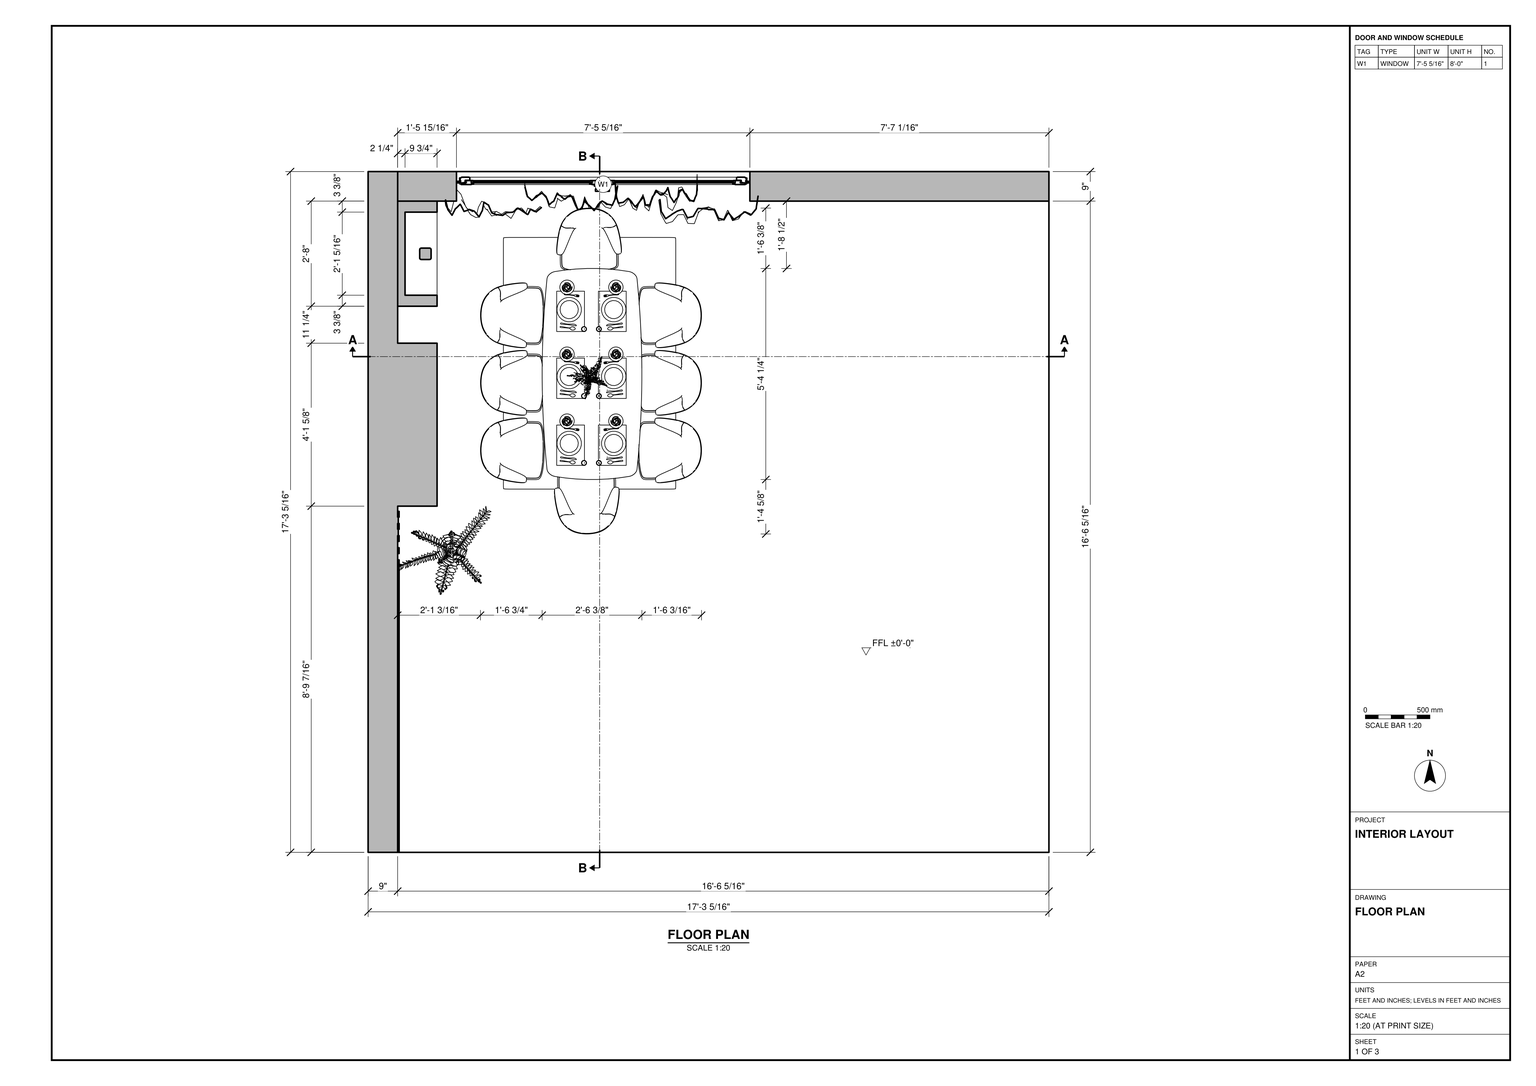
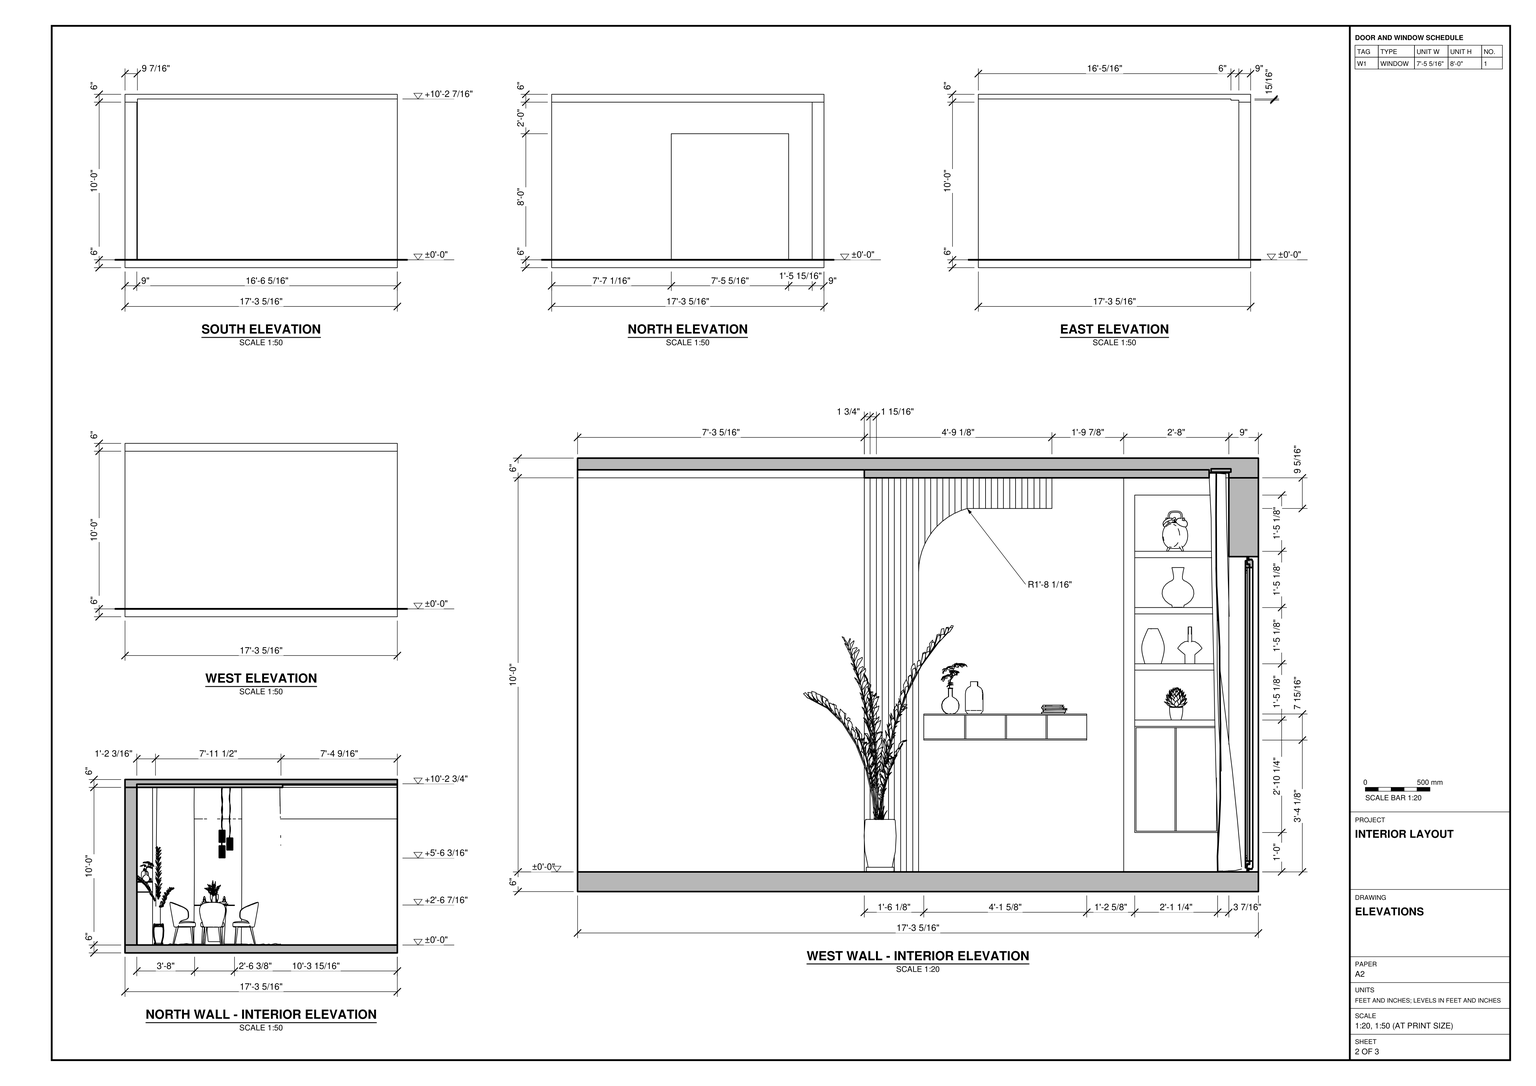
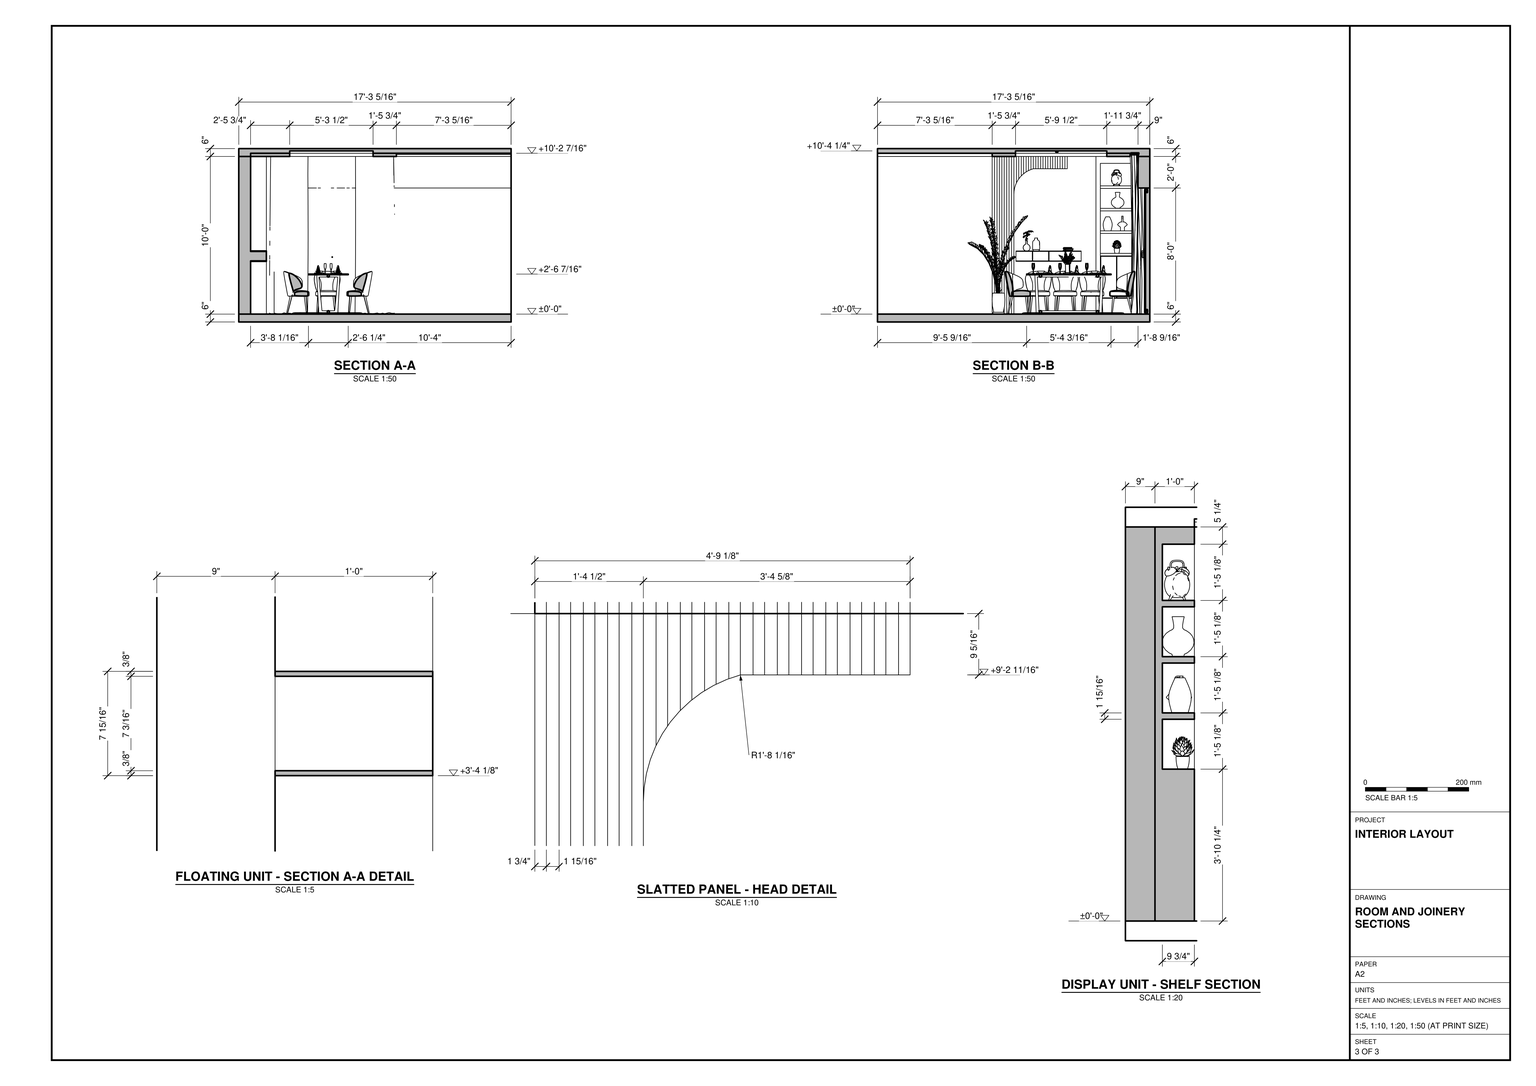
Build the dining room in SketchUp using task_files/diagram_01.pdf. Work in feet and inches. The overall footprint is 17'-3 5/16" by 17'-3 5/16", the overall height is 11'-0", and the finished floor level is ±0'-0". Model the floor slab, the 9" north and west walls and the overhead slab. Follow the sections for the slab thicknesses and changes in the ceiling profile. Leave the south and east sides open as drawn.

Place the floor-height window and curtains near the west end of the north wall. Set the dining table with its long axis running north–south in front of the window. Arrange three chairs along each long side and one at each end, with the rug beneath the setting and pendant lighting above it.

Use the west wall elevation and joinery details to model the vertical slats and their curved return into a horizontal head. Fit the shallow floating unit beside the slats and the tall display unit nearer the window. Include the display shelves, lower cabinet and loose items in the positions shown. Decor and loose items may be any suitable library components.

Keep the walls, slabs and each furniture or joinery piece in separate groups or components, and use components for repeated parts. Save one SketchUp model as output_files/dining_room_with_slatted_panelling_and_display_joinery.skp.

# SketchUp Ruby script. Lengths in inches.
U = 1.inch
M = Sketchup.active_model
def pt(a) = Geom::Point3d.new(a.map { |v| v * U })
def face(e, loops, mat)
  f = e.add_face(loops[0].map { |a| pt(a) })
  loops[1..].each { |l| e.add_face(l.map { |a| pt(a) }).erase! }
  f.material = f.back_material = mat if mat
  f
end
# faces: each face lists its corners as indices into pts; further lists are holes
def faces(e, pts, list, mat = nil) = list.each { |f| face(e, (f[0].is_a?(Array) ? f : [f]).map { |l| l.map { |i| pts[i] } }, mat) }
# xy, xz, yz: faces in a plane at the given z, y or x. An outline is a flat list of corners, or four numbers for a rectangle; further outlines are holes
def ring(l) = l.size == 4 ? [[l[0], l[1]], [l[2], l[1]], [l[2], l[3]], [l[0], l[3]]] : l.each_slice(2).to_a
def flat(e, list, mat, &to3) = list.each { |f| face(e, (f[0].is_a?(Array) ? f : [f]).map { |l| ring(l).map { |u, v| to3.(u, v) } }, mat) }
def xy(e, z, list, mat = nil) = flat(e, list, mat) { |x, y| [x, y, z] }
def xz(e, y, list, mat = nil) = flat(e, list, mat) { |x, z| [x, y, z] }
def yz(e, x, list, mat = nil) = flat(e, list, mat) { |y, z| [x, y, z] }
def lines(e, pts, list) = list.each { |a, b| e.add_line(pt(pts[a]), pt(pts[b])) }
# prism: a flat outline (further loops are holes) pulled along v
def prism(e, loops, v, mat = nil)
  f = face(e, loops, mat); d = Geom::Vector3d.new(v.map { |x| x * U })
  f.pushpull(f.normal.samedirection?(d) ? d.length : -d.length)
end
def box(e, o, s, mat = nil) = prism(e, [[o, [o[0] + s[0], o[1], o[2]], [o[0] + s[0], o[1] + s[1], o[2]], [o[0], o[1] + s[1], o[2]]]], [0, 0, s[2]], mat)
def at(x, y, z, deg = 0) = Geom::Transformation.translation(pt([x, y, z])) * Geom::Transformation.rotation(ORIGIN, Z_AXIS, deg.degrees)
def axes(o, x, y, z) = Geom::Transformation.new([*x, 0, *y, 0, *z, 0, *pt(o).to_a, 1])
def part(name) = M.definitions.add(name)
# library, detail: a bought-in or finely detailed component or shape, given as its bounding box
def library(name, o, s) = part(name).tap { |d| box(d.entities, o, s) }
def detail(e, o, s) = box(e.add_group.entities, o, s)
def put(e, d, t, mat = nil) = e.add_instance(d, t).tap { |i| i.material = mat if mat }
def group(e, t, mat = nil) = e.add_group.tap { |g| g.transformation = t; g.material = mat if mat }.entities
root = M.entities
M.materials.add("Emissive").color = [224, 222, 181]
M.materials.add("[Color M01]").color = [226, 226, 226]
M.materials.add("[Color M03]").color = [179, 160, 140]
M.materials.add("[Color M05]").color = [114, 114, 114]
M.materials.add("[Wood Floor]").color = [155, 105, 61]
c1 = library("Window 46-12",[-37.28,-2.15,0],[74.56,4.3,92.91])
c2 = library("Curtains 001",[-91.88,-6.87,0.16],[183.71,15.03,109.46])
c3 = library("Dining Table",[-4.14,-4.14,0],[95.74,137.21,49.0625])
c4 = library("Rug 293 007",[-90.2,-61.78,-0.71],[180.4,123.56,1.82])
c5 = library("Potted Plant 02",[-16.98,-19.78,0],[30.04,38.68,37.52])
c6 = library("Vase 111-18",[-4.54,-2.8,0.01],[10.64,7.87,15.5])
c7 = library("Vase 010",[-2.69,-2.69,0.01],[5.38,5.38,9.84])
c8 = library("Vase 20-10",[-4.83,-4.83,0],[9.66,9.66,14.63])
c9 = library("Ornamental Vase 001",[-3.84,-3.66,0],[7.68,7.32,10.13])
c10 = library("Vase 298 004 008",[-3.43,-3.43,-0.03],[6.86,6.87,9.09])
c11 = library("Alarm Clock 114 007",[-2.86,-1.17,0.01],[5.71,2.99,7.86])
c12 = library("Potted Plant 50-23",[-3.4,-3.5,0],[6.8,7,9.93])
c13 = library("Books 193 006",[-5.22,-3.55,0],[10.44,7.83,2.69])
c14 = library("Pendant 35-41",[-5.93,-5.84,-58.05],[11.88,11.67,58.05])
xy(root,-6,[[0,0,207.3125,207.3125]])
xy(root,0,[[0,0,0,207.3125,9,207.3125,9,102.08,9.1875,102.08,9.1875,100.14,9,100.14,9,98.39,9.1875,98.39,9.1875,96.45,9,96.45,9,0],[9,0,9.4375,87.3125],[9,87.3125,9.4375,89.07],[9,91,9.4375,92.76],[9,94.7,9.4375,96.45],
  [9,98.39,9.4375,100.14],[9,102.08,9.4375,103.84],[9,166.3,21,198.3125],[9,198.3125,26.91,207.3125],[116.25,198.3125,207.3125,207.3125]])
xy(root,0,[[9.4375,0,207.3125,0,207.3125,198.3125,116.25,198.3125,116.25,207.3125,26.91,207.3125,26.91,198.3125,21,198.3125,21,166.3,9,166.3,9,103.84,9.4375,103.84,9.4375,102.08,9.1875,102.08,9.1875,100.14,9.4375,100.14,9.4375,98.39,9.1875,98.39,9.1875,96.45,9.4375,96.45,9.4375,94.7,9,94.7,9,92.76,9.4375,92.76,9.4375,91,9,91,9,89.07,9.4375,89.07]],"[Color M05]")
xy(root,40.14,[[9,105.42,10,155.05],[10,105.42,21,155.05]])
xy(root,40.52,[[9,105.42,21,155.05]])
xy(root,46.25,[[11.25,169.66,21,194.96]])
xy(root,47.7,[[9,105.42,21,155.05]])
xy(root,48.08,[[9,105.42,21,155.05]])
xy(root,61.4375,[[12.25,169.66,21,194.96]])
xy(root,61.4375,[[11.25,169.66,12.25,194.96]],"Emissive")
xy(root,63.375,[[11.25,169.66,21,194.96]],"[Color M05]")
xy(root,78.5625,[[12.25,169.66,21,194.96]])
xy(root,78.5625,[[11.25,169.66,12.25,194.96]],"Emissive")
xy(root,80.5,[[11.25,169.66,21,194.96]])
xy(root,95.6875,[[11.25,169.66,12.25,194.96]],"Emissive")
xy(root,95.6875,[[12.25,169.66,21,194.96]],"[Color M05]")
xy(root,96,[[26.91,198.3125,116.25,207.3125]])
xy(root,97.625,[[11.25,169.66,21,194.96]])
xy(root,110.66,[[9,118.6,9.1875,120.54],[9,120.54,9.4375,122.29],[9,122.29,9.1875,124.23],[9,124.23,9.4375,125.99],[9,125.99,9.1875,127.92],
  [9,127.92,9.4375,129.68],[9,129.68,9.1875,131.61],[9,131.61,9.4375,133.37],[9,133.37,9.1875,135.3],[9,135.3,9.4375,137.0625],
  [9,137.0625,9.1875,139],[9,139,9.4375,140.75],[9,140.75,9.1875,142.6875],[9,142.6875,9.4375,144.44]],"Emissive")
xy(root,114.75,[[11.25,169.66,12.25,194.96]],"Emissive")
xy(root,114.75,[[12.25,169.66,21,194.96]],"[Color M05]")
xy(root,120,[[0,0,0,207.3125,9,207.3125,9,142.6875,9.1875,142.6875,9.1875,140.75,9,140.75,9,139,9.1875,139,9.1875,137.0625,9,137.0625,9,135.3,9.1875,135.3,9.1875,133.37,9,133.37,9,131.61,9.1875,131.61,9.1875,129.68,9,129.68,9,127.92,9.1875,127.92,9.1875,125.99,9,125.99,9,124.23,9.1875,124.23,9.1875,122.29,9,122.29,9,120.54,9.1875,120.54,9.1875,118.6,9,118.6,9,116.85,9.1875,116.85,9.1875,114.91,9,114.91,9,113.15,9.1875,113.15,9.1875,111.22,9,111.22,9,109.46,9.1875,109.46,9.1875,107.53,9,107.53,9,105.77,9.1875,105.77,9.1875,103.84,9,103.84,9,102.08,9.1875,102.08,9.1875,100.14,9,100.14,9,98.39,9.1875,98.39,9.1875,96.45,9,96.45,9,0],[9,0,9.4375,87.3125],[9,87.3125,9.4375,89.07],[9,91,9.4375,92.76],[9,94.7,9.4375,96.45],
  [9,98.39,9.4375,100.14],[9,102.08,9.4375,103.84],[9,105.77,9.4375,107.53],[9,109.46,9.4375,111.22],[9,113.15,9.4375,114.91],
  [9,116.85,9.4375,118.6],[9,120.54,9.4375,122.29],[9,124.23,9.4375,125.99],[9,127.92,9.4375,129.68],[9,131.61,9.4375,133.37],
  [9,135.3,9.4375,137.0625],[9,139,9.4375,140.75],[9,142.6875,9.4375,144.44],[9,166.3,21,198.3125],[9,198.3125,207.3125,207.3125]])
xy(root,120,[[[9.4375,87.3125,9.4375,89.07,9,89.07,9,91,9.4375,91,9.4375,92.76,9,92.76,9,94.7,9.4375,94.7,9.4375,96.45,9.1875,96.45,9.1875,98.39,9.4375,98.39,9.4375,100.14,9.1875,100.14,9.1875,102.08,9.4375,102.08,9.4375,103.84,9.1875,103.84,9.1875,105.77,9.4375,105.77,9.4375,107.53,9.1875,107.53,9.1875,109.46,9.4375,109.46,9.4375,111.22,9.1875,111.22,9.1875,113.15,9.4375,113.15,9.4375,114.91,9.1875,114.91,9.1875,116.85,9.4375,116.85,9.4375,118.6,9.1875,118.6,9.1875,120.54,9.4375,120.54,9.4375,122.29,9.1875,122.29,9.1875,124.23,9.4375,124.23,9.4375,125.99,9.1875,125.99,9.1875,127.92,9.4375,127.92,9.4375,129.68,9.1875,129.68,9.1875,131.61,9.4375,131.61,9.4375,133.37,9.1875,133.37,9.1875,135.3,9.4375,135.3,9.4375,137.0625,9.1875,137.0625,9.1875,139,9.4375,139,9.4375,140.75,9.1875,140.75,9.1875,142.6875,9.4375,142.6875,9.4375,144.44,9,144.44,9,166.3,21,166.3,21,192.3125,120,192.3125,120,87.3125],[38.76,105.07,102.24,174.55]]],"[Color M01]")
xy(root,121.5,[[21,192.3125,207.3125,198.3125]])
xy(root,122.4375,[[9.4375,0,120,87.3125],[120,0,207.3125,192.3125],[[9.4375,87.3125,120,87.3125,120,192.3125,21,192.3125,21,166.3,9,166.3,9,144.44,9.4375,144.44,9.4375,142.6875,9.1875,142.6875,9.1875,140.75,9,140.75,9,139,9.1875,139,9.1875,137.0625,9,137.0625,9,135.3,9.1875,135.3,9.1875,133.37,9,133.37,9,131.61,9.1875,131.61,9.1875,129.68,9,129.68,9,127.92,9.1875,127.92,9.1875,125.99,9,125.99,9,124.23,9.1875,124.23,9.1875,122.29,9,122.29,9,120.54,9.1875,120.54,9.1875,118.6,9,118.6,9,116.85,9.1875,116.85,9.1875,114.91,9,114.91,9,113.15,9.1875,113.15,9.1875,111.22,9,111.22,9,109.46,9.1875,109.46,9.1875,107.53,9,107.53,9,105.77,9.1875,105.77,9.1875,103.84,9,103.84,9,102.08,9.1875,102.08,9.1875,100.14,9,100.14,9,98.39,9.1875,98.39,9.1875,96.45,9,96.45,9,89.07,9.4375,89.07],[38.76,105.07,102.24,174.55]]])
xy(root,124.25,[[38.76,105.07,102.24,174.55]])
xy(root,126,[[0,0,207.3125,207.3125]])
xz(root,0,[[0,-6,207.3125,0],[0,0,9,120],[9,0,9.4375,120],[9.4375,0,207.3125,122.4375],[0,120,9.4375,120,9.4375,122.4375,207.3125,122.4375,207.3125,126,0,126]])
xz(root,87.3125,[[9,0,9.4375,120],[9.4375,120,120,122.4375]])
xz(root,89.07,[[9,120,9.4375,122.4375]])
xz(root,89.07,[[9,0,9.4375,120]],"[Wood Floor]")
xz(root,91,[[9,0,9.4375,120]],"[Wood Floor]")
xz(root,92.76,[[9,0,9.4375,120]],"[Wood Floor]")
xz(root,94.7,[[9,0,9.4375,120]],"[Wood Floor]")
xz(root,96.45,[[9,0,9.1875,120],[9,120,9.1875,122.4375]])
xz(root,96.45,[[9.1875,0,9.4375,120]],"[Wood Floor]")
xz(root,98.39,[[9,0,9.1875,120],[9,120,9.1875,122.4375]])
xz(root,98.39,[[9.1875,0,9.4375,120]],"[Wood Floor]")
xz(root,100.14,[[9,0,9.1875,120],[9,120,9.1875,122.4375]])
xz(root,100.14,[[9.1875,0,9.4375,120]],"[Wood Floor]")
xz(root,102.08,[[9,0,9.1875,120],[9,120,9.1875,122.4375]])
xz(root,102.08,[[9.1875,0,9.4375,120]],"[Wood Floor]")
xz(root,103.84,[[9,91.35,9.1875,120],[9.1875,91.35,9.4375,120],[9,120,9.1875,122.4375]])
xz(root,103.84,[[9,0,9.4375,91.35]],"[Wood Floor]")
xz(root,105.07,[[38.76,120,102.24,122.4375]])
xz(root,105.07,[[38.76,122.4375,102.24,124.25]],"Emissive")
xz(root,105.42,[[9,40.14,21,40.52],[9,47.7,21,48.08]])
xz(root,105.42,[[9,40.52,21,47.7]],"[Color M05]")
xz(root,105.77,[[9,99.91,9.1875,120],[9.1875,99.91,9.4375,120],[9,120,9.1875,122.4375]])
xz(root,107.53,[[9,102.88,9.1875,120],[9.1875,102.88,9.4375,120],[9,120,9.1875,122.4375]])
xz(root,109.46,[[9,105.25,9.1875,120],[9.1875,105.25,9.4375,120],[9,120,9.1875,122.4375]])
xz(root,111.22,[[9,106.85,9.1875,120],[9.1875,106.85,9.4375,120],[9,120,9.1875,122.4375]])
xz(root,113.15,[[9,108.24,9.1875,120],[9.1875,108.24,9.4375,120],[9,120,9.1875,122.4375]])
xz(root,114.91,[[9,109.24,9.1875,120],[9.1875,109.24,9.4375,120],[9,120,9.1875,122.4375]])
xz(root,116.85,[[9,110.08,9.1875,120],[9.1875,110.08,9.4375,120],[9,120,9.1875,122.4375]])
xz(root,118.6,[[9,110.66,9.1875,120],[9.1875,110.66,9.4375,120],[9,120,9.1875,122.4375]])
xz(root,120.54,[[9,110.66,9.1875,120],[9.1875,110.66,9.4375,120],[9,120,9.1875,122.4375]])
xz(root,122.29,[[9,110.66,9.1875,120],[9.1875,110.66,9.4375,120],[9,120,9.1875,122.4375]])
xz(root,124.23,[[9,110.66,9.1875,120],[9.1875,110.66,9.4375,120],[9,120,9.1875,122.4375]])
xz(root,125.99,[[9,110.66,9.1875,120],[9.1875,110.66,9.4375,120],[9,120,9.1875,122.4375]])
xz(root,127.92,[[9,110.66,9.1875,120],[9.1875,110.66,9.4375,120],[9,120,9.1875,122.4375]])
xz(root,129.68,[[9,110.66,9.1875,120],[9.1875,110.66,9.4375,120],[9,120,9.1875,122.4375]])
xz(root,131.61,[[9,110.66,9.1875,120],[9.1875,110.66,9.4375,120],[9,120,9.1875,122.4375]])
xz(root,133.37,[[9,110.66,9.1875,120],[9.1875,110.66,9.4375,120],[9,120,9.1875,122.4375]])
xz(root,135.3,[[9,110.66,9.1875,120],[9.1875,110.66,9.4375,120],[9,120,9.1875,122.4375]])
xz(root,137.0625,[[9,110.66,9.1875,120],[9.1875,110.66,9.4375,120],[9,120,9.1875,122.4375]])
xz(root,139,[[9,110.66,9.1875,120],[9.1875,110.66,9.4375,120],[9,120,9.1875,122.4375]])
xz(root,140.75,[[9,110.66,9.1875,120],[9.1875,110.66,9.4375,120],[9,120,9.1875,122.4375]])
xz(root,142.6875,[[9,110.66,9.1875,120],[9.1875,110.66,9.4375,120],[9.1875,120,9.4375,122.4375]])
xz(root,144.44,[[9,110.66,9.4375,120],[9,120,9.4375,122.4375]])
xz(root,155.05,[[9,40.14,21,40.52],[9,40.52,21,47.7],[9,47.7,21,48.08]])
xz(root,166.3,[[9,120,21,122.4375]])
xz(root,166.3,[[9,0,21,120]],"[Color M05]")
xz(root,169.66,[[11.25,46.25,21,61.4375],[11.25,63.375,21,78.5625],[11.25,80.5,21,95.6875],[11.25,97.625,21,114.75]])
xz(root,174.55,[[38.76,120,102.24,122.4375]])
xz(root,174.55,[[38.76,122.4375,102.24,124.25]],"Emissive")
xz(root,192.3125,[[21,120,120,121.5],[21,121.5,120,122.4375],[120,121.5,207.3125,122.4375]])
xz(root,194.96,[[11.25,46.25,21,61.4375],[11.25,63.375,21,78.5625],[11.25,80.5,21,95.6875],[11.25,97.625,21,114.75]],"[Color M05]")
xz(root,198.3125,[[9,0,21,120],[21,0,26.91,0,26.91,96,207.3125,96,207.3125,120,21,120],[116.25,0,207.3125,96],[21,120,207.3125,121.5]])
xz(root,207.3125,[[0,-6,207.3125,0],[0,0,9,120],[9,0,9,120,207.3125,120,207.3125,0,116.25,0,116.25,96,26.91,96,26.91,0],[26.91,0,116.25,96],[0,120,207.3125,126]])
yz(root,0,[[0,-6,207.3125,0],[0,0,207.3125,120],[0,120,207.3125,126]])
yz(root,9,[[0,0,87.3125,120],[87.3125,0,89.07,120],[91,0,92.76,120],[94.7,0,96.45,120],[98.39,0,100.14,120],
  [102.08,0,103.84,120],[166.3,0,198.3125,120],[198.3125,0,207.3125,120],[105.42,40.14,155.05,40.52],[105.42,47.7,155.05,48.08],
  [105.77,99.91,105.77,120,107.53,120,107.53,102.88,106.73,101.71],[109.46,105.25,109.46,120,111.22,120,111.22,106.85,110.95,106.65],[113.15,108.24,113.15,120,114.91,120,114.91,109.24,114.56,109.07],[116.85,110.08,116.85,120,118.6,120,118.6,110.66],[120.54,110.66,122.29,120],
  [124.23,110.66,125.99,120],[127.92,110.66,129.68,120],[131.61,110.66,133.37,120],[135.3,110.66,137.0625,120],[139,110.66,140.75,120],
  [142.6875,110.66,144.44,120],[89.07,120,91,122.4375],[91,120,92.76,122.4375],[92.76,120,94.7,122.4375],[94.7,120,96.45,122.4375],
  [98.39,120,100.14,122.4375],[102.08,120,103.84,122.4375],[105.77,120,107.53,122.4375],[109.46,120,111.22,122.4375],[113.15,120,114.91,122.4375],
  [116.85,120,118.6,122.4375],[120.54,120,122.29,122.4375],[124.23,120,125.99,122.4375],[127.92,120,129.68,122.4375],[131.61,120,133.37,122.4375],
  [135.3,120,137.0625,122.4375],[139,120,140.75,122.4375],[144.44,120,166.3,122.4375]])
yz(root,9,[[[103.84,0,166.3,0,166.3,120,144.44,120,144.44,110.66,118.6,110.66,116.85,110.08,116.54,109.98,114.91,109.24,114.56,109.07,113.15,108.24,112.6875,107.96,111.22,106.85,110.95,106.65,109.46,105.25,109.36,105.16,107.95,103.5,107.53,102.88,106.73,101.71,105.77,99.91,105.7,99.78,104.89,97.76,104.31,95.67,103.95,93.52,103.84,91.35],[105.42,40.14,155.05,48.08]]],"[Color M03]")
yz(root,9,[[89.07,0,91,120],[92.76,0,94.7,120]],"[Wood Floor]")
yz(root,9.1875,[[96.45,120,98.39,122.4375],[100.14,120,102.08,122.4375],[103.84,120,105.77,122.4375],[107.53,120,109.46,122.4375],[111.22,120,113.15,122.4375],
  [114.91,120,116.85,122.4375],[118.6,120,120.54,122.4375],[122.29,120,124.23,122.4375],[125.99,120,127.92,122.4375],[129.68,120,131.61,122.4375],
  [133.37,120,135.3,122.4375],[137.0625,120,139,122.4375],[140.75,120,142.6875,122.4375]])
yz(root,9.1875,[[96.45,0,98.39,120],[100.14,0,102.08,120],[103.84,91.35,103.95,93.52,104.31,95.67,104.89,97.76,105.7,99.78,105.77,99.91,105.77,120,103.84,120],[107.53,102.88,107.95,103.5,109.36,105.16,109.46,105.25,109.46,120,107.53,120],[111.22,106.85,112.6875,107.96,113.15,108.24,113.15,120,111.22,120],
  [114.91,109.24,116.54,109.98,116.85,110.08,116.85,120,114.91,120],[118.6,110.66,120.54,120],[122.29,110.66,124.23,120],[125.99,110.66,127.92,120],[129.68,110.66,131.61,120],
  [133.37,110.66,135.3,120],[137.0625,110.66,139,120],[140.75,110.66,142.6875,120]],"[Wood Floor]")
yz(root,9.4375,[[0,0,87.3125,120],[0,120,87.3125,122.4375],[87.3125,120,89.07,122.4375],[142.6875,120,144.44,122.4375]])
yz(root,9.4375,[[87.3125,0,89.07,120],[91,0,92.76,120],[94.7,0,96.45,120],[98.39,0,100.14,120],[102.08,0,103.84,120],
  [105.77,99.91,106.73,101.71,107.53,102.88,107.53,120,105.77,120],[109.46,105.25,110.95,106.65,111.22,106.85,111.22,120,109.46,120],[113.15,108.24,114.56,109.07,114.91,109.24,114.91,120,113.15,120],[116.85,110.08,118.6,110.66,118.6,120,116.85,120],[120.54,110.66,122.29,120],
  [124.23,110.66,125.99,120],[127.92,110.66,129.68,120],[131.61,110.66,133.37,120],[135.3,110.66,137.0625,120],[139,110.66,140.75,120],
  [142.6875,110.66,144.44,120]],"[Wood Floor]")
yz(root,11.25,[[169.66,46.25,194.96,61.4375],[169.66,63.375,194.96,78.5625],[169.66,80.5,194.96,95.6875],[169.66,97.625,194.96,114.75]],"[Color M05]")
yz(root,21,[[[169.66,12,194.96,44.3125],[170.06,12.4,194.5625,43.91]],[181.91,12.4,182.31,43.91],[105.42,40.14,155.05,40.52],[117.83,40.52,118.23,47.7],[130.24,40.52,130.64,47.7],
  [142.64,40.52,143.04,47.7],[105.42,47.7,155.05,48.08],[166.3,120,192.3125,122.4375],[192.3125,120,198.3125,121.5]])
yz(root,21,[[[166.3,0,198.3125,120],[169.66,12,194.96,114.75]],[170.06,12.4,181.91,43.91],[182.31,12.4,194.5625,43.91],[105.42,40.52,117.83,47.7],[118.23,40.52,130.24,47.7],
  [130.64,40.52,142.64,47.7],[143.04,40.52,155.05,47.7],[169.66,44.3125,194.96,46.25],[169.66,61.4375,194.96,63.375],[169.66,78.5625,194.96,80.5],
  [169.66,95.6875,194.96,97.625]],"[Color M05]")
yz(root,26.91,[[198.3125,0,207.3125,96]])
yz(root,38.76,[[105.07,120,174.55,122.4375]])
yz(root,38.76,[[105.07,122.4375,174.55,124.25]],"Emissive")
yz(root,102.24,[[105.07,120,174.55,122.4375]])
yz(root,102.24,[[105.07,122.4375,174.55,124.25]],"Emissive")
yz(root,116.25,[[198.3125,0,207.3125,96]])
yz(root,120,[[87.3125,120,192.3125,122.4375]])
yz(root,207.3125,[[0,-6,207.3125,0],[0,0,198.3125,0,198.3125,121.5,192.3125,121.5,192.3125,122.4375,0,122.4375],[198.3125,0,207.3125,120],[198.3125,120,207.3125,120,207.3125,126,0,126,0,122.4375,192.3125,122.4375,192.3125,121.5,198.3125,121.5]])
p = [[9,103.84,91.35],[9,103.95,93.52],[9.1875,103.95,93.52],[9.1875,103.84,91.35],[9,104.31,95.67],[9.1875,104.31,95.67],
  [9,104.89,97.76],[9.1875,104.89,97.76],[9,105.7,99.78],[9.1875,105.7,99.78],[9,105.77,99.91],[9.1875,105.77,99.91],
  [9,106.73,101.71],[9.4375,106.73,101.71],[9.4375,105.77,99.91],[9,107.53,102.88],[9.1875,107.53,102.88],[9.4375,107.53,102.88],
  [9,107.95,103.5],[9.1875,107.95,103.5],[9,109.36,105.16],[9.1875,109.36,105.16],[9,109.46,105.25],[9.1875,109.46,105.25],
  [9,110.95,106.65],[9.4375,110.95,106.65],[9.4375,109.46,105.25],[9,111.22,106.85],[9.1875,111.22,106.85],[9.4375,111.22,106.85],
  [9,112.6875,107.96],[9.1875,112.6875,107.96],[9,113.15,108.24],[9.1875,113.15,108.24],[9,114.56,109.07],[9.4375,114.56,109.07],
  [9.4375,113.15,108.24],[9,114.91,109.24],[9.1875,114.91,109.24],[9.4375,114.91,109.24],[9,116.54,109.98],[9.1875,116.54,109.98],
  [9,116.85,110.08],[9.1875,116.85,110.08],[9,118.6,110.66],[9.1875,118.6,110.66],[9.4375,118.6,110.66],[9.4375,116.85,110.08],
  [11.25,195.96,114.75],[11.25,194.96,114.75],[12.25,195.96,114.75],[12.25,194.96,114.75]]
faces(root,p,[[0,1,2,3],[1,4,5,2],[4,6,7,5],[6,8,9,7],[8,10,11,9],[10,12,13,14,11],[12,15,16,17,13],[15,18,19,16],
  [18,20,21,19],[20,22,23,21],[22,24,25,26,23],[24,27,28,29,25],[27,30,31,28],[30,32,33,31],[32,34,35,36,33],[34,37,38,39,35],
  [37,40,41,38],[40,42,43,41],[42,44,45,46,47,43]],"Emissive")
lines(root,p,[[48,49],[50,51]])
put(root,c1,axes([71.58,203.46,0],[1.19808,0,0],[0,1,0],[0,0,1.03322]))
put(root,c2,axes([70.99,198.3125,-0.02],[0.52,0,0],[0,1,0],[0,0,1.12]))
put(root,c3,axes([34.2,96.93,0],[0.77,0,0],[0,0.77,0],[0,0,1]))
put(root,c4,axes([67.43,148.94,0.3],[0,-0.4248,0],[0.4248,0,0],[0,0,0.4248]))
put(root,c5,axes([25.53,92.13,0],[1.07,0,0],[0,1.18,0],[0,0,2]))
put(root,c6,at(16.01,113.52,48.08))
put(root,c7,at(15.1,120.77,48.08))
put(root,c8,axes([16.05,182.83,80.5],[1,0,0],[0,1,0],[0,0,0.833]))
put(root,c9,axes([16.32,186.45,63.375],[1,0,0],[0,1,0],[0,0,1.11]))
put(root,c10,axes([16.61,175.23,63.38],[1,0,0],[0,1,0],[0,0,1.18]))
put(root,c11,axes([15.74,181.96,97.62],[1.10309,1.10309,0],[-1.10309,1.10309,0],[0,0,1.56]))
put(root,c12,at(17.48,182.125,46.25))
put(root,c13,at(15.23,144.8,48.08))
put(root,c14,at(76.28,136.53,124.25))
